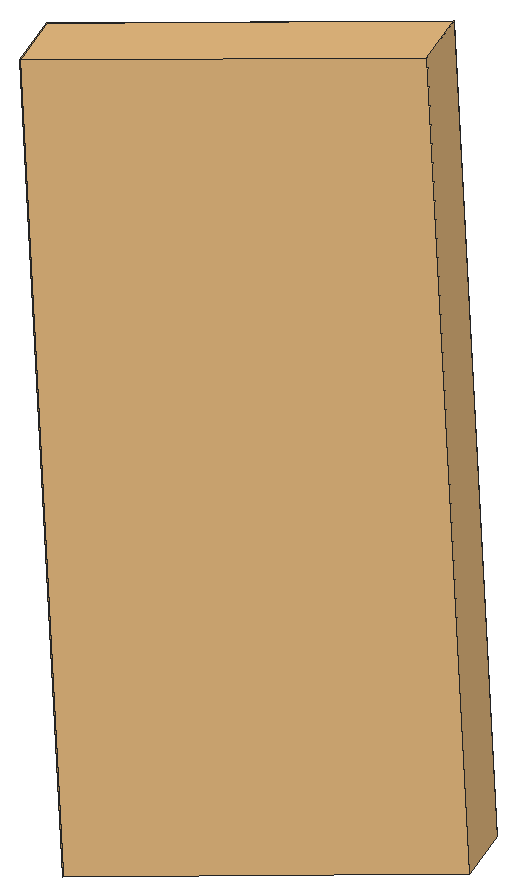
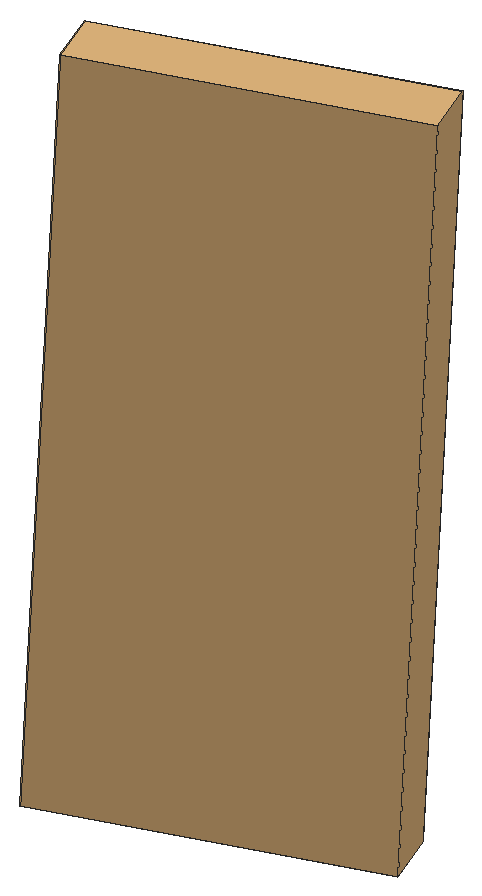
# SketchUp Ruby script. Lengths in inches.
U = 1.inch
M = Sketchup.active_model
def pt(a) = Geom::Point3d.new(a.map { |v| v * U })
def face(e, loops, mat)
  f = e.add_face(loops[0].map { |a| pt(a) })
  loops[1..].each { |l| e.add_face(l.map { |a| pt(a) }).erase! }
  f.material = f.back_material = mat if mat
  f
end
# faces: each face lists its corners as indices into pts; further lists are holes
def faces(e, pts, list, mat = nil) = list.each { |f| face(e, (f[0].is_a?(Array) ? f : [f]).map { |l| l.map { |i| pts[i] } }, mat) }
# xy, xz, yz: faces in a plane at the given z, y or x. An outline is a flat list of corners, or four numbers for a rectangle; further outlines are holes
def ring(l) = l.size == 4 ? [[l[0], l[1]], [l[2], l[1]], [l[2], l[3]], [l[0], l[3]]] : l.each_slice(2).to_a
def flat(e, list, mat, &to3) = list.each { |f| face(e, (f[0].is_a?(Array) ? f : [f]).map { |l| ring(l).map { |u, v| to3.(u, v) } }, mat) }
def xy(e, z, list, mat = nil) = flat(e, list, mat) { |x, y| [x, y, z] }
def xz(e, y, list, mat = nil) = flat(e, list, mat) { |x, z| [x, y, z] }
def yz(e, x, list, mat = nil) = flat(e, list, mat) { |y, z| [x, y, z] }
def lines(e, pts, list) = list.each { |a, b| e.add_line(pt(pts[a]), pt(pts[b])) }
# prism: a flat outline (further loops are holes) pulled along v
def prism(e, loops, v, mat = nil)
  f = face(e, loops, mat); d = Geom::Vector3d.new(v.map { |x| x * U })
  f.pushpull(f.normal.samedirection?(d) ? d.length : -d.length)
end
def box(e, o, s, mat = nil) = prism(e, [[o, [o[0] + s[0], o[1], o[2]], [o[0] + s[0], o[1] + s[1], o[2]], [o[0], o[1] + s[1], o[2]]]], [0, 0, s[2]], mat)
def at(x, y, z, deg = 0) = Geom::Transformation.translation(pt([x, y, z])) * Geom::Transformation.rotation(ORIGIN, Z_AXIS, deg.degrees)
def axes(o, x, y, z) = Geom::Transformation.new([*x, 0, *y, 0, *z, 0, *pt(o).to_a, 1])
def part(name) = M.definitions.add(name)
# library, detail: a bought-in or finely detailed component or shape, given as its bounding box
def library(name, o, s) = part(name).tap { |d| box(d.entities, o, s) }
def detail(e, o, s) = box(e.add_group.entities, o, s)
def put(e, d, t, mat = nil) = e.add_instance(d, t).tap { |i| i.material = mat if mat }
def group(e, t, mat = nil) = e.add_group.tap { |g| g.transformation = t; g.material = mat if mat }.entities
root = M.entities
c1 = library("sm2 st v2 Component\#1",[0,0,0],[29.46,4.93,43.46])
put(root,c1,axes([83.72,102.65,71.17],[-0.37738,-0.20211,-0.04675],[0.16326,-0.46967,-0.00077],[-0.02678,-0.015,0.65403]))
